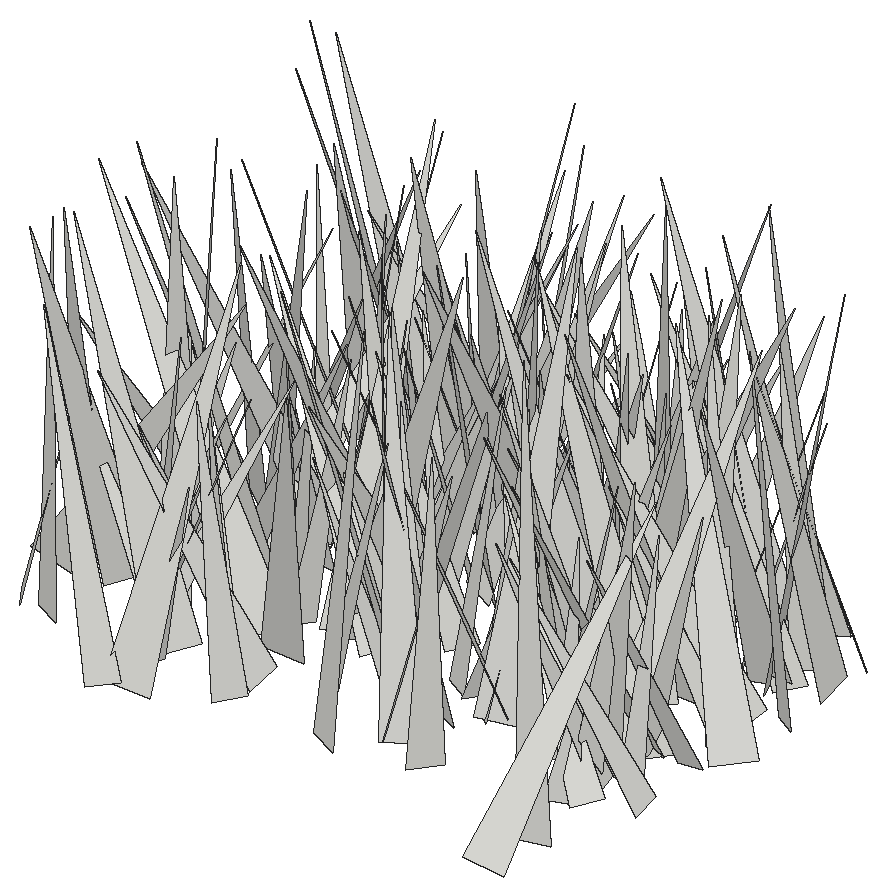
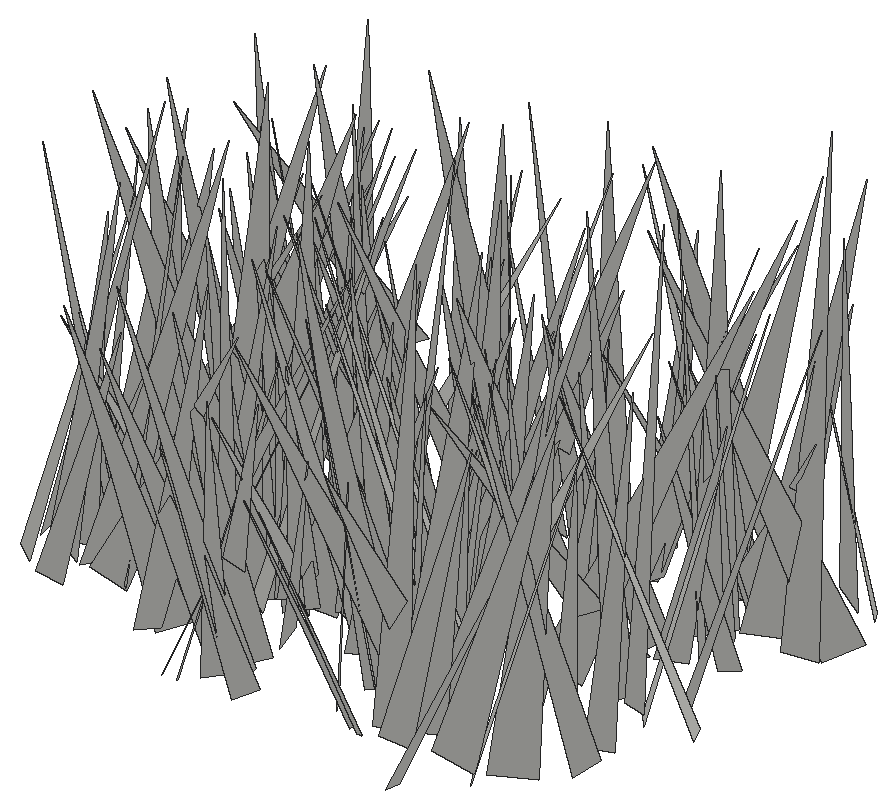
# SketchUp Ruby script. Lengths in inches.
U = 1.inch
M = Sketchup.active_model
def pt(a) = Geom::Point3d.new(a.map { |v| v * U })
def face(e, loops, mat)
  f = e.add_face(loops[0].map { |a| pt(a) })
  loops[1..].each { |l| e.add_face(l.map { |a| pt(a) }).erase! }
  f.material = f.back_material = mat if mat
  f
end
# faces: each face lists its corners as indices into pts; further lists are holes
def faces(e, pts, list, mat = nil) = list.each { |f| face(e, (f[0].is_a?(Array) ? f : [f]).map { |l| l.map { |i| pts[i] } }, mat) }
# xy, xz, yz: faces in a plane at the given z, y or x. An outline is a flat list of corners, or four numbers for a rectangle; further outlines are holes
def ring(l) = l.size == 4 ? [[l[0], l[1]], [l[2], l[1]], [l[2], l[3]], [l[0], l[3]]] : l.each_slice(2).to_a
def flat(e, list, mat, &to3) = list.each { |f| face(e, (f[0].is_a?(Array) ? f : [f]).map { |l| ring(l).map { |u, v| to3.(u, v) } }, mat) }
def xy(e, z, list, mat = nil) = flat(e, list, mat) { |x, y| [x, y, z] }
def xz(e, y, list, mat = nil) = flat(e, list, mat) { |x, z| [x, y, z] }
def yz(e, x, list, mat = nil) = flat(e, list, mat) { |y, z| [x, y, z] }
def lines(e, pts, list) = list.each { |a, b| e.add_line(pt(pts[a]), pt(pts[b])) }
# prism: a flat outline (further loops are holes) pulled along v
def prism(e, loops, v, mat = nil)
  f = face(e, loops, mat); d = Geom::Vector3d.new(v.map { |x| x * U })
  f.pushpull(f.normal.samedirection?(d) ? d.length : -d.length)
end
def box(e, o, s, mat = nil) = prism(e, [[o, [o[0] + s[0], o[1], o[2]], [o[0] + s[0], o[1] + s[1], o[2]], [o[0], o[1] + s[1], o[2]]]], [0, 0, s[2]], mat)
def at(x, y, z, deg = 0) = Geom::Transformation.translation(pt([x, y, z])) * Geom::Transformation.rotation(ORIGIN, Z_AXIS, deg.degrees)
def axes(o, x, y, z) = Geom::Transformation.new([*x, 0, *y, 0, *z, 0, *pt(o).to_a, 1])
def part(name) = M.definitions.add(name)
# library, detail: a bought-in or finely detailed component or shape, given as its bounding box
def library(name, o, s) = part(name).tap { |d| box(d.entities, o, s) }
def detail(e, o, s) = box(e.add_group.entities, o, s)
def put(e, d, t, mat = nil) = e.add_instance(d, t).tap { |i| i.material = mat if mat }
def group(e, t, mat = nil) = e.add_group.tap { |g| g.transformation = t; g.material = mat if mat }.entities
root = M.entities
c1 = part("fur_instance\#9")
p = [[0.8125,0,1.79],[0.67,-0.02,1.48],[0,-0.11,0],[0,0.11,0]]
faces(c1.entities,p,[[0,1,2,3]])
put(root,c1,axes([93.54,413.52,-27.1],[-1.50811,5.89701,0.63499],[5.61901,1.21081,2.10069],[-1.89858,-1.1007,5.71281]))
put(root,c1,axes([110.04,411.91,-27.1],[-2.9172,5.75801,0.16061],[5.28877,2.74872,-2.48273],[2.2824,0.99014,5.95825]))
put(root,c1,axes([97.21,415.26,-27.1],[-4.02078,2.93374,1.78068],[3.22926,4.16274,0.43339],[1.1617,-1.41743,4.95839]))
put(root,c1,axes([93.89,415.61,-27.1],[3.66443,-1.25509,0.51627],[-1.25966,-3.69872,-0.05095],[-0.50503,0.11865,3.87307]))
put(root,c1,axes([94.28,413.79,-27.1],[-1.25446,7.26591,1.58891],[7.27727,1.53186,-1.25954],[1.53602,-1.32352,7.26503]))
put(root,c1,axes([104.67,415.7,-27.1],[4.30224,-3.16543,2.15858],[-3.43037,-4.62804,0.05027],[-1.70646,1.32286,5.34104]))
put(root,c1,axes([97.22,416.94,-27.1],[-5.99784,0.36822,0.31916],[0.44096,5.77868,1.61988],[0.20737,-1.63795,5.78668]))
put(root,c1,axes([110.3,414.05,-27.1],[0.70044,7.59304,1.85976],[7.56257,-1.13109,1.76971],[-1.98005,-1.63401,7.41708]))
put(root,c1,axes([93.37,414.75,-27.1],[3.56009,0.21869,0.65734],[0.01468,-3.46445,1.07311],[-0.69261,1.05069,3.40155]))
put(root,c1,axes([101.21,414.95,-27.1],[3.25616,5.95918,2.11371],[6.15078,-3.5363,0.49462],[-1.46542,-1.60155,6.77272]))
put(root,c1,axes([88.04,416.32,-27.1],[3.15545,2.01724,0.79775],[2.15051,-3.09372,-0.68323],[-0.2846,-1.01105,3.6823]))
put(root,c1,axes([93.95,416.64,-27.1],[-6.02527,4.37662,1.94606],[4.73834,5.90349,1.39383],[0.70004,-2.28907,7.31546]))
put(root,c1,axes([96.71,418.52,-27.1],[1.84605,-6.6162,0.27609],[-6.51912,-1.76548,1.28157],[1.16252,0.60597,6.74831]))
put(root,c1,axes([92.05,418.23,-27.1],[6.81977,1.54998,0.06465],[1.44583,-6.24479,-2.79788],[0.56233,-2.74155,6.40965]))
put(root,c1,axes([102.37,416.625,-27.1],[3.27913,1.40298,0.59687],[1.4938,-3.23974,-0.59158],[-0.30522,-0.78299,3.51725]))
put(root,c1,axes([89.36,415.97,-27.1],[3.04497,5.63186,2.55497],[5.93211,-3.46487,0.56775],[-1.7481,-1.94792,6.3771]))
put(root,c1,axes([111.65,418.02,-27.1],[-4.90231,-0.23018,0.15933],[-0.18525,4.76264,1.18065],[0.20988,-1.17272,4.76358]))
put(root,c1,axes([109.8125,418.23,-27.1],[-4.7933,-0.97536,0.74224],[-0.77682,4.73507,1.20565],[0.94805,-1.05153,4.74061]))
put(root,c1,axes([95.92,416.74,-27.1],[-4.49863,-0.46507,1.40367],[-0.60193,4.68178,-0.37796],[1.35065,0.53749,4.50678]))
put(root,c1,axes([89.95,419.36,-27.1],[5.20163,-5.29224,1.8402],[-4.95757,-5.51713,-1.85336],[-2.61089,-0.0677,7.18539]))
put(root,c1,axes([94.8,418.69,-27.1],[-4.25051,-1.02119,0.70994],[-0.79222,4.17184,1.25768],[0.95876,-1.08007,4.18663]))
put(root,c1,axes([88.28,419.73,-27.1],[-1.25565,-8.18969,1.33935],[-8.04493,1.53362,1.83538],[2.03567,1.00923,8.07955]))
put(root,c1,axes([103.15,416.48,-27.1],[-2.95923,6.17255,1.7602],[6.41346,2.92118,0.53848],[0.25723,-1.82266,6.82403]))
put(root,c1,axes([103.28,418.46,-27.1],[-2.87551,-4.98025,1.4124],[-5.17006,2.84441,-0.49611],[0.26119,1.47404,5.72934]))
put(root,c1,axes([98.9,418.29,-27.1],[3.06956,3.90435,1.71137],[4.25532,-2.68017,-1.51785],[0.25498,-2.27325,4.72887]))
put(root,c1,axes([110.06,417.07,-27.1],[-3.00277,4.1066,0.06153],[3.92812,2.84936,1.52829],[-1.19912,-0.94951,4.85234]))
put(root,c1,axes([109.02,419.01,-27.1],[1.26894,-6.32164,1.3833],[-6.3592,-0.957,1.46001],[1.19887,1.6149,6.28026]))
put(root,c1,axes([109.34,417.8,-27.1],[4.20018,-2.603,1.54886],[-2.85846,-4.28223,0.55487],[-1.0019,1.30501,4.91012]))
put(root,c1,axes([92.45,417.33,-27.1],[4.52412,1.43506,1.852],[1.32361,-4.8885,0.5546],[-1.93323,0.01133,4.71375]))
put(root,c1,axes([92.18,418.05,-27.1],[-2.52559,2.65872,0.46687],[2.62617,2.27215,1.26725],[-0.62447,-1.19747,3.44114]))
put(root,c1,axes([95.65,417.19,-27.1],[-3.44021,1.49763,0.22694],[1.46636,3.43395,-0.43273],[0.37973,0.30751,3.72702]))
put(root,c1,axes([107.625,419.05,-27.1],[-1.75963,-5.21212,1.71135],[-5.46295,1.82898,-0.04671],[0.50104,1.63703,5.50093]))
put(root,c1,axes([101.33,418.78,-27.1],[-5.74367,-4.09689,1.01684],[-4.21686,5.6466,-1.0688],[0.19121,1.46278,6.97366]))
put(root,c1,axes([109.2,416.54,-27.1],[-3.77654,1.99621,0.89861],[1.50689,3.67022,-1.82025],[1.58796,1.26459,3.86442]))
put(root,c1,axes([87.36,418.74,-27.1],[3.63581,-6.29578,1.08718],[-5.74464,-2.67402,3.72648],[2.79605,2.69271,6.24254]))
put(root,c1,axes([90.93,418.79,-27.1],[2.90459,3.11145,0.76807],[3.13189,-2.53582,-1.57117],[0.67994,-1.61126,3.9559]))
put(root,c1,axes([107.38,418.88,-27.1],[4.01593,3.70117,1.52807],[3.99587,-3.8439,-1.19115],[-0.25835,-1.92018,5.32987]))
put(root,c1,axes([109.5,420.9375,-27.1],[-1.38983,-5.84462,0.0201],[-5.82782,1.38425,-0.46046],[-0.44334,0.12603,5.98992]))
put(root,c1,axes([107.8,418.7,-27.1],[0.95056,-3.70171,1.6828],[-4.06505,-0.90725,0.30052],[-0.09921,1.70654,3.80998]))
put(root,c1,axes([92.52,417.35,-27.1],[1.65691,4.63189,0.02775],[4.518,-1.60961,-1.09423],[1.0212,-0.39403,4.79608]))
put(root,c1,axes([100.51,419.1875,-27.1],[-3.97846,-0.22397,0.26493],[-0.21326,3.98441,0.16592],[0.27363,-0.15114,3.9813]))
put(root,c1,axes([101.83,419.15,-27.1],[-1.39517,3.65073,1.37856],[3.73252,0.82124,1.60268],[-1.13865,-1.78115,3.56451]))
put(root,c1,axes([95.36,419.24,-27.1],[-7.15301,3.97515,0.71331],[4.02795,6.91641,1.848],[-0.2937,-1.95899,7.97197]))
put(root,c1,axes([111.08,420.95,-27.1],[-0.25255,-4.7231,0.0991],[-4.68784,0.23828,-0.59045],[-0.58449,0.12972,4.69284]))
put(root,c1,axes([110.53,418.67,-27.1],[0.04059,4.23783,1.33242],[4.44047,0.00019,-0.13586],[0.12965,-1.33303,4.23585]))
put(root,c1,axes([107.43,417.43,-27.1],[1.37607,4.21587,0.41156],[3.82506,-1.42264,1.78368],[-1.81985,0.19763,4.06025]))
put(root,c1,axes([104.52,419.98,-27.1],[-5.23491,-4.53939,0.15815],[-4.43832,5.06084,-1.65066],[-0.96564,1.34804,6.72946]))
put(root,c1,axes([101.74,418.95,-27.1],[-4.02288,2.74208,1.38872],[2.85785,4.17888,0.02734],[1.13147,-0.80565,4.86845]))
put(root,c1,axes([106.97,420.83,-27.1],[3.89618,-1.88557,1.1779],[-1.51971,-3.99347,-1.36592],[-1.62275,-0.78732,4.1073]))
put(root,c1,axes([91.29,420.26,-27.1],[6.49174,-3.69034,2.54193],[-3.75607,-6.92147,-0.45599],[-2.44375,0.83512,7.45341]))
put(root,c1,axes([108.35,420.47,-27.1],[-6.30832,-1.1114,1.05664],[-1.00602,6.37534,0.69964],[1.15742,-0.51611,6.36715]))
put(root,c1,axes([92.85,418.13,-27.1],[-4.63028,1.37895,0.71291],[1.15549,4.55932,-1.31404],[1.03661,1.07721,4.64912]))
put(root,c1,axes([108.73,420.92,-27.1],[-1.67937,-5.43767,0.87836],[-5.25266,1.30456,-1.96667],[-1.65811,1.37475,5.34049]))
put(root,c1,axes([99.68,420.62,-27.1],[3.13596,-3.23192,0.2957],[-3.22644,-3.06024,0.76944],[0.35051,0.74607,4.43707]))
put(root,c1,axes([97.97,420.8,-27.1],[6.25642,-5.32962,1.03257],[-5.42827,-6.12142,1.29455],[0.06986,1.65444,8.11614]))
put(root,c1,axes([98.69,423.33,-27.1],[5.3138,-2.81187,1.14067],[-1.98861,-4.96443,-2.9739],[-2.29198,-2.2118,5.22484]))
put(root,c1,axes([104.12,419.29,-27.1],[2.60004,3.22909,0.64132],[3.22546,-2.66223,0.32783],[-0.65933,-0.2899,4.13277]))
put(root,c1,axes([98.32,422.99,-27.1],[-0.28332,-7.79704,0.77926],[-7.68212,0.12267,-1.56569],[-1.54472,0.82004,7.64347]))
put(root,c1,axes([109.55,420.5,-27.1],[4.23339,-1.74729,1.15695],[-1.93705,-4.25778,0.65751],[-0.79963,1.0637,4.53236]))
put(root,c1,axes([99.19,420.59,-27.1],[4.97701,4.02381,2.97396],[4.34378,-5.5566,0.24873],[-2.48337,-1.65505,6.3953]))
put(root,c1,axes([94.78,420.7,-27.1],[-7.32124,-3.15954,0.71739],[-3.23761,7.2018,-1.32279],[0.12329,1.49974,7.86343]))
put(root,c1,axes([95.95,420.41,-27.1],[4.38322,-1.64948,1.59394],[-1.93146,-4.50849,0.64578],[-1.2373,1.19448,4.63858]))
put(root,c1,axes([104.78,419.4,-27.1],[-2.78975,7.45432,2.27613],[7.61508,3.12201,-0.8911],[1.66081,-1.79348,7.90921]))
put(root,c1,axes([105.29,420.04,-27.1],[-1.61358,3.38665,0.61033],[3.4322,1.63258,0.01498],[0.24881,-0.55751,3.75138]))
put(root,c1,axes([88.97,424.53,-27.1],[-5.2943,-3.28141,1.0592],[-2.29433,4.80125,3.40634],[2.57403,-2.46971,5.21479]))
put(root,c1,axes([102.29,420.25,-27.1],[2.52877,4.50107,1.40807],[4.66336,-2.62485,0.01569],[-0.70386,-1.21962,5.16276]))
put(root,c1,axes([102.89,421.92,-27.1],[3.51068,-4.45404,1.06123],[-4.56743,-3.50052,0.41776],[-0.32136,1.09429,5.65587]))
put(root,c1,axes([99.51,421.69,-27.1],[1.40139,-5.88916,2.09043],[-6.21682,-1.53152,-0.14692],[-0.635,1.99706,6.05182]))
put(root,c1,axes([103.08,420.1875,-27.1],[5.00649,-0.69371,1.01239],[-0.92226,-4.93206,1.18126],[-0.80969,1.32843,4.91435]))
put(root,c1,axes([98.99,420.67,-27.1],[-4.99082,4.3261,0.4502],[4.29852,4.80129,1.51542],[-0.66378,-1.43477,6.4286]))
put(root,c1,axes([94.99,421.5,-27.1],[-3.86454,-2.68359,1.87384],[-2.96857,4.09497,-0.25773],[1.3786,1.29506,4.69786]))
put(root,c1,axes([109.89,420.72,-27.1],[-2.9065,7.574,1.65107],[7.44857,2.24028,2.83534],[-2.14716,-2.4809,7.60092]))
put(root,c1,axes([90.45,421.83,-27.1],[6.26613,3.81902,2.82967],[4.24719,-6.60086,-0.4964],[-2.13385,-1.92357,7.3214]))
put(root,c1,axes([90.23,420.76,-27.1],[-4.86729,-1.78674,2.25978],[-2.35287,5.02555,-1.09424],[1.66225,1.88173,5.06809]))
put(root,c1,axes([94.93,421.37,-27.1],[4.11345,0.18865,1.81103],[0.00918,-4.47631,0.44541],[-1.8208,0.4036,4.09361]))
put(root,c1,axes([89.45,421.75,-27.1],[0.33455,3.97904,1.71347],[4.11253,0.24873,-1.38056],[1.36232,-1.72801,3.74683]))
put(root,c1,axes([92.24,421.9375,-27.1],[4.93305,-2.19664,0.15391],[-2.18894,-4.85066,0.92924],[0.23965,0.9109,5.31946]))
put(root,c1,axes([108.61,424.14,-27.1],[-0.93689,-7.58778,0.99671],[-7.63501,0.85799,-0.64504],[-0.52389,1.06539,7.61814]))
put(root,c1,axes([100.84,422.375,-27.1],[-3.29735,3.76242,1.32483],[3.9802,2.99017,1.41439],[-0.2628,-1.92005,4.79874]))
put(root,c1,axes([110.91,422.9,-27.1],[-4.62797,0.36048,0.06702],[0.36662,4.56134,0.78248],[0.00509,-0.78533,4.57556]))
put(root,c1,axes([108.73,419.96,-27.1],[-1.75958,6.89289,0.89816],[6.66639,1.93582,-1.79628],[1.96924,-0.39424,6.88342]))
put(root,c1,axes([100.51,419.7,-27.1],[7.12647,2.20024,1.82821],[1.44023,-6.99989,2.8102],[-2.47167,2.26505,6.90872]))
put(root,c1,axes([106.92,422.46,-27.1],[-8.06825,0.70999,0.37952],[0.71569,8.07597,0.10667],[0.36866,-0.13964,8.09873]))
put(root,c1,axes([94.24,423.71,-27.1],[-0.05824,-3.81958,0.55077],[-3.85535,0.08183,0.15984],[0.16986,0.54776,3.81668]))
put(root,c1,axes([102.33,423.4,-27.1],[7.07527,1.73735,2.55738],[2.12787,-7.36989,-0.88027],[-2.24293,-1.5114,7.23207]))
put(root,c1,axes([91.21,422.44,-27.1],[-3.33055,3.67395,0.98734],[3.8043,3.21801,0.85849],[0.0046,-1.30837,4.884]))
put(root,c1,axes([103.05,422.7,-27.1],[1.88047,-2.78184,1.95652],[-3.20631,-2.19563,-0.04014],[-1.13412,1.59479,3.35756]))
put(root,c1,axes([112.04,421.89,-27.1],[-4.84886,5.21937,0.60309],[5.25064,4.78392,0.8135],[-0.19034,-0.99462,7.07753]))
put(root,c1,axes([110.8,424.27,-27.1],[-6.49837,1.01991,0.13564],[1.01971,6.26851,1.71854],[-0.13717,-1.71841,6.34946]))
put(root,c1,axes([104.99,423.11,-27.1],[4.67154,-2.82363,0.84685],[-2.94301,-4.55853,1.0353],[-0.16964,1.32674,5.35951]))
put(root,c1,axes([93.52,425.01,-27.1],[0.24896,-7.3468,1.55373],[-6.97419,-0.80255,-2.67734],[-2.78393,1.35351,6.84612]))
put(root,c1,axes([104.75,425.08,-27.1],[-0.95692,-4.60949,0.0097],[-4.59629,0.95343,-0.35816],[-0.34872,0.08227,4.69412]))
put(root,c1,axes([89.56,425.88,-27.1],[-5.06426,-4.56399,0.84014],[-4.29824,5.08189,1.69768],[1.74956,-0.72593,6.60262]))
put(root,c1,axes([102.01,426.72,-27.1],[1.8393,-7.94223,0.20343],[-7.82957,-1.84746,-1.33722],[-1.34842,-0.10629,8.04201]))
put(root,c1,axes([90.24,425.47,-27.1],[-3.33298,-6.74445,1.96036],[-6.484,3.7887,2.01069],[2.69971,0.77298,7.24938]))
put(root,c1,axes([99.2,425.76,-27.1],[-3.9717,-6.10655,1.7462],[-5.81347,4.32471,1.90107],[2.55787,0.34722,7.03209]))
put(root,c1,axes([107.67,423.125,-27.1],[-5.36752,5.77658,2.45123],[6.12108,5.53013,0.37117],[1.38195,-2.05828,7.87664]))
put(root,c1,axes([98.78,423.57,-27.1],[-0.11529,-4.79427,2.44231],[-5.06003,0.9271,1.58106],[1.8292,2.26244,4.52754]))
put(root,c1,axes([90.97,425.34,-27.1],[7.66875,0.29762,1.40281],[0.64374,-7.5341,-1.92071],[-1.28143,-2.00373,7.43029]))
put(root,c1,axes([102.77,421.22,-27.1],[3.19327,6.60837,0.52108],[6.51338,-3.23542,1.11669],[-1.23207,0.02336,7.254]))
put(root,c1,axes([95.83,423.9,-27.1],[3.79573,2.84609,1.46317],[3.05532,-3.89817,-0.34352],[-0.95191,-1.16307,4.73179]))
put(root,c1,axes([111.21,422.53,-27.1],[-0.8728,6.82324,1.17968],[6.78553,0.6058,1.51645],[-1.38016,-1.33658,6.7096]))
put(root,c1,axes([109.79,426.58,-27.1],[2.0561,-6.44135,0.2848],[-6.4395,-2.06652,-0.24899],[-0.32395,0.19535,6.75697]))
put(root,c1,axes([105.97,424.36,-27.1],[7.40162,-2.04644,1.37858],[-2.14984,-7.48787,0.42713],[-1.21103,0.78507,7.66743]))
put(root,c1,axes([101.21,426.48,-27.1],[0.94954,-6.1364,0.24208],[-6.03443,-0.88683,1.18943],[1.14,0.41683,6.09444]))
put(root,c1,axes([96.5,424.83,-27.1],[-4.53938,3.59005,2.40826],[4.08452,4.7056,0.68422],[1.41595,-2.06469,5.74685]))
put(root,c1,axes([96.81,424.44,-27.1],[-5.69424,-4.56861,0.52497],[-4.47673,5.31586,-2.29625],[-1.05201,2.10752,6.92992]))
put(root,c1,axes([103.17,426.95,-27.1],[-1.64763,-7.14584,1.34901],[-6.49832,2.06763,3.01567],[3.26416,0.50931,6.68457]))
put(root,c1,axes([99.08,425.26,-27.1],[-3.66395,-2.75565,0.79106],[-2.79858,3.7164,-0.01609],[0.62239,0.48852,4.58453]))
put(root,c1,axes([97.39,420.81,-27.1],[-7.03666,4.34174,0.35439],[3.96979,6.66848,-2.87454],[1.79361,2.2741,7.75256]))
put(root,c1,axes([102.15,427.02,-27.1],[0.44147,-7.17503,0.62576],[-6.54369,-0.13768,3.03788],[3.00878,0.75334,6.51516]))
put(root,c1,axes([103.5,426.67,-27.1],[2.17041,-4.52553,0.56409],[-4.42394,-2.24099,-0.95709],[-1.10786,0.0828,4.92697]))
put(root,c1,axes([106.53,425.3,-27.1],[-5.73495,-0.11109,1.68244],[-0.04447,5.97258,0.24275],[1.68552,-0.22038,5.73089]))
put(root,c1,axes([111.72,424.86,-27.1],[-3.6941,-4.73944,2.34113],[-5.23892,3.66336,-0.85037],[0.70493,2.38895,5.94858]))
put(root,c1,axes([108.33,424.79,-27.1],[4.86014,-4.74094,2.82615],[-5.30574,-5.05065,0.65171],[-1.52079,2.46963,6.75816]))
put(root,c1,axes([101.46,424.8,-27.1],[-3.65531,3.57205,1.42816],[3.77376,3.712,0.37448],[0.74692,-1.27356,5.09712]))
put(root,c1,axes([102.6,426.45,-27.1],[4.53182,-5.76132,1.66498],[-5.89155,-4.66684,-0.11276],[-1.12014,1.237,7.32923]))
put(root,c1,axes([103.43,427.58,-27.1],[-4.06699,-5.2197,0.56162],[-5.13541,4.10303,0.94539],[1.09007,-0.14467,6.54919]))
put(root,c1,axes([95.58,423.93,-27.1],[-5.55203,-0.57439,2.02149],[-1.15794,5.60149,-1.58866],[1.75372,1.88009,5.3508]))
put(root,c1,axes([97.56,424.86,-27.1],[-5.21816,-1.76906,1.50642],[-2.07355,5.2165,-1.05669],[1.04846,1.51216,5.4076]))
put(root,c1,axes([104.67,426.67,-27.1],[1.53942,-5.44162,0.89342],[-5.38829,-1.28703,1.44538],[1.17292,1.22946,5.46735]))
put(root,c1,axes([98.83,428.02,-27.1],[4.29462,-4.11505,0.26594],[-3.98176,-4.23808,-1.27765],[-1.07236,-0.74374,5.80905]))
put(root,c1,axes([87.69,425.57,-27.1],[5.0651,3.0377,0.15182],[3.00547,-4.95362,-1.15532],[0.46672,-1.0677,5.79207]))
put(root,c1,axes([100.43,426.71,-27.1],[-1.57238,-4.56901,1.11948],[-4.65933,1.35009,-1.0341],[-0.64787,1.37945,4.72005]))
put(root,c1,axes([89.45,428.2,-27.1],[-0.0268,-5.65268,0.22398],[-5.53849,0.07185,1.15049],[1.15241,0.21383,5.53443]))
put(root,c1,axes([103.93,426.76,-27.1],[6.6749,-4.96789,0.00129],[-4.8195,-6.47499,2.02019],[1.20515,1.62135,8.07174]))
put(root,c1,axes([92.21,423.23,-27.1],[-1.93127,6.17376,0.09606],[5.65668,1.80943,-2.5656],[2.47519,0.68189,5.93825]))
put(root,c1,axes([96.31,426.62,-27.1],[3.07396,-3.53335,0.83024],[-3.61315,-2.87553,1.13994],[0.34489,1.36741,4.5425]))
put(root,c1,axes([110.48,426.6875,-27.1],[-2.9134,4.03937,1.46912],[4.26943,2.51447,1.5531],[-0.49677,-2.07934,4.73205]))
put(root,c1,axes([94.87,427.2,-27.1],[7.11507,4.33314,0.48127],[4.20256,-6.57141,-2.9643],[1.16029,-2.76992,7.78545]))
put(root,c1,axes([111.57,427.5,-27.1],[-7.78363,-1.77881,1.5879],[-1.77027,7.9428,0.22014],[1.59741,0.13482,7.98126]))
put(root,c1,axes([108.25,427.13,-27.1],[4.56554,2.4835,0.72557],[2.58092,-4.47494,-0.92307],[-0.18188,-1.15993,5.11467]))
put(root,c1,axes([96.28,427.02,-27.1],[1.74245,-3.02379,2.07472],[-3.3962,-2.19711,-0.34987],[-1.38332,1.58534,3.47232]))
put(root,c1,axes([98.14,427.5,-27.1],[-0.07815,-6.05054,2.52953],[-6.4447,0.53908,1.09033],[1.2138,2.47266,5.952]))
put(root,c1,axes([102.42,426.51,-27.1],[-3.32764,3.062,1.30373],[3.08153,3.53122,-0.42827],[1.25687,-0.55083,4.50173]))
put(root,c1,axes([92.98,426.41,-27.1],[4.79862,3.05458,1.6678],[3.017,-5.06719,0.60002],[-1.73486,-0.36311,5.65661]))
put(root,c1,axes([109.79,426.53,-27.1],[6.18065,2.99725,1.89028],[2.99834,-6.44896,0.42186],[-1.88855,-0.42956,6.85609]))
put(root,c1,axes([104.9,427.9,-27.1],[-2.89308,-3.13599,0.85003],[-3.23039,2.89836,-0.3018],[0.34876,0.83187,4.25597]))
put(root,c1,axes([108.58,424.99,-27.1],[4.22042,3.02936,0.44277],[2.70703,-4.0447,1.87014],[-1.43005,1.2839,4.84681]))
put(root,c1,axes([105.48,428.98,-27.1],[-6.50951,0.22142,0.60358],[0.38251,6.26967,1.82536],[0.51674,-1.85181,6.25226]))
put(root,c1,axes([93.46,425.1,-27.1],[5.52585,4.05046,1.31825],[3.69086,-5.63091,1.83015],[-2.12639,0.75214,6.60241]))
put(root,c1,axes([97.21,428.14,-27.1],[2.58883,2.26123,2.35644],[2.87323,-3.00647,-0.27159],[-1.55259,-1.79333,3.42658]))
put(root,c1,axes([99.04,425.39,-27.1],[3.08355,6.47581,0.56476],[6.50039,-3.07095,-0.27862],[0.00972,-0.62967,7.16706]))
put(root,c1,axes([97.79,425.65,-27.1],[6.38887,5.18246,1.59043],[5.07791,-6.58181,1.04866],[-1.89794,-0.16426,8.1594]))
put(root,c1,axes([111.0625,429.53,-27.1],[-3.86726,-4.8383,0.71579],[-4.78645,3.93151,0.71436],[1.00566,0.10641,6.1526]))
put(root,c1,axes([110.19,428.03,-27.1],[1.93856,-5.12728,2.24723],[-5.46022,-2.25638,-0.43794],[-1.23493,1.9279,5.46399]))
put(root,c1,axes([107.72,428.86,-27.1],[4.54557,4.08977,3.87164],[5.12111,-5.0718,-0.65499],[-2.34307,-3.15097,6.07942]))
put(root,c1,axes([99.33,427.37,-27.1],[6.39922,1.66084,0.77373],[1.68967,-6.43637,-0.15871],[-0.70856,-0.34898,6.60932]))
put(root,c1,axes([94.66,429.43,-27.1],[-4.58981,-6.81856,1.14154],[-6.9132,4.53833,-0.68805],[0.05895,1.33156,8.19058]))
put(root,c1,axes([92.05,426.58,-27.1],[1.02305,5.31057,1.33507],[5.15193,-1.39366,1.59576],[-1.8553,-0.94167,5.16743]))
put(root,c1,axes([108.83,428.37,-27.1],[-7.81883,2.51294,1.68172],[2.76611,7.82758,1.16397],[1.22135,-1.64052,8.12983]))
put(root,c1,axes([96.57,429.13,-27.1],[-2.51428,-3.3921,0.48717],[-3.39486,2.54791,0.21985],[0.4675,0.25907,4.21659]))
put(root,c1,axes([94.82,428.4,-27.1],[6.0574,2.72005,0.2303],[2.69232,-5.86042,-1.5971],[0.45071,-1.54939,6.44516]))
put(root,c1,axes([94.48,430.8,-27.1],[5.05065,-5.78899,0.88016],[-5.66798,-5.12516,-1.18448],[-1.47008,-0.1285,7.59069]))
put(root,c1,axes([96.73,428.47,-27.1],[4.08139,-3.20586,0.61223],[-3.2526,-3.91407,1.18774],[0.27008,1.30866,5.05219]))
put(root,c1,axes([96.99,429.28,-27.1],[1.53835,-7.01276,2.03333],[-7.04829,-0.88366,2.28484],[1.90652,2.39168,6.80623]))
put(root,c1,axes([96,429.28,-27.1],[-2.86919,-3.90872,1.79506],[-4.01549,3.2075,0.56601],[1.54149,1.08002,4.8156]))
put(root,c1,axes([90.48,431.18,-27.1],[4.1786,-6.03386,0.40804],[-6.0035,-4.19846,-0.60465],[-0.72937,-0.01047,7.31455]))
put(root,c1,axes([102.89,429.67,-27.1],[7.08469,1.17747,2.52447],[1.61288,-7.35894,-1.094],[-2.27113,-1.55299,7.09806]))
put(root,c1,axes([91.4,430.97,-27.1],[-2.96228,-3.48582,0.87467],[-2.85625,2.97145,2.16874],[2.18125,-0.843,4.02773]))
put(root,c1,axes([102.74,429.43,-27.1],[3.92592,-0.41216,0.89749],[-0.2951,-4.00034,-0.54626],[-0.94248,-0.46433,3.90952]))
put(root,c1,axes([110.44,428.39,-27.1],[1.97558,6.78512,3.04566],[6.89111,-2.85534,1.89119],[-2.79761,-2.24188,6.80913]))
put(root,c1,axes([102.38,426.31,-27.1],[4.15865,3.49208,0.81847],[2.77358,-3.92559,2.6563],[-2.27416,1.59814,4.73636]))
put(root,c1,axes([95.24,431.23,-27.1],[-0.53699,-7.34105,1.16615],[-7.27133,0.76139,1.44476],[1.5423,1.0337,7.21748]))
put(root,c1,axes([89,429.37,-27.1],[6.32916,0.13104,0.27334],[0.13733,-6.3333,-0.14369],[-0.27023,-0.14945,6.32889]))
put(root,c1,axes([108.02,429.2,-27.1],[-2.44299,5.49091,1.30941],[5.27932,1.71736,2.64808],[-1.99837,-2.17564,5.395]))
put(root,c1,axes([109.48,430.3,-27.1],[0.38107,-4.3176,1.24457],[-4.35966,-0.65774,-0.94692],[-1.08815,1.12319,4.22969]))
put(root,c1,axes([101.37,428.66,-27.1],[-4.4304,-0.23548,0.66281],[-0.42328,4.26855,-1.31284],[0.56178,1.35914,4.23796]))
put(root,c1,axes([101.25,430.52,-27.1],[4.31446,-3.71791,0.40504],[-3.72385,-4.21342,0.9907],[0.3462,1.01276,5.60856]))
put(root,c1,axes([97.84,428.84,-27.1],[-4.49953,-3.59508,3.80394],[-4.60675,5.10137,-0.62788],[2.48443,2.94818,5.72505]))
put(root,c1,axes([104.97,430.76,-27.1],[4.62611,-3.05223,2.53258],[-2.97331,-5.24406,-0.88892],[-2.62479,0.5609,5.47054]))
put(root,c1,axes([102.95,429.93,-27.1],[1.4221,-3.78822,2.5832],[-4.25079,-2.10312,-0.74405],[-1.71882,2.06693,3.97736]))
put(root,c1,axes([103.09,432.61,-27.1],[-4.66281,-2.88259,0.04543],[-2.761,4.48988,1.50703],[0.82963,-1.25893,5.27068]))
put(root,c1,axes([95.04,429.53,-27.1],[6.3813,-2.25892,0.20905],[-2.20352,-6.02357,2.17449],[0.53935,2.11689,6.41056]))
put(root,c1,axes([102.64,430.36,-27.1],[3.58397,-3.64133,0.7361],[-3.60405,-3.15993,1.91614],[0.90107,1.84433,4.7363]))
put(root,c1,axes([94.66,431.73,-27.1],[0.91416,-4.94391,1.27953],[-4.9749,-1.15567,-0.91103],[-1.1532,1.06645,4.94449]))
put(root,c1,axes([102.39,432.84,-27.1],[-3.17214,-2.54983,0.51656],[-2.07776,2.97317,1.9168],[1.56569,-1.22048,3.59026]))
put(root,c1,axes([97.56,430.97,-27.1],[2.96101,1.91002,1.7712],[2.18546,-3.28075,-0.11568],[-1.41742,-1.06838,3.5217]))
put(root,c1,axes([104.51,430.3125,-27.1],[3.63193,-4.05591,1.60644],[-4.34601,-3.18259,1.79036],[0.37856,2.37544,5.14159]))
put(root,c1,axes([95.87,428.18,-27.1],[-4.47907,3.89554,0.463],[3.44419,4.24137,-2.36643],[1.87807,1.51235,5.44401]))
put(root,c1,axes([96.32,431.77,-27.1],[2.45066,3.05169,0.44917],[2.65928,-1.79957,-2.28257],[1.56295,-1.7231,3.17938]))
put(root,c1,axes([101.59,431.92,-27.1],[3.58428,-2.61771,1.24135],[-2.70899,-3.7283,-0.04015],[-1.02701,0.69843,4.43823]))
put(root,c1,axes([92.49,431.6,-27.1],[0.18988,-6.4583,3.19895],[-6.79344,-1.22898,-2.07794],[-2.40669,2.95955,6.11783]))
put(root,c1,axes([91.7,431.5,-27.1],[-6.3033,-3.29184,1.05702],[-3.45211,6.11366,-1.54635],[0.19083,1.86335,6.94094]))
put(root,c1,axes([100.15,432.25,-27.1],[3.34433,-2.45993,0.06359],[-2.39384,-3.22746,1.0454],[0.56992,0.87868,4.01783]))
put(root,c1,axes([100.78,431.55,-27.1],[6.76067,1.19839,0.69108],[1.18973,-6.79585,0.14582],[-0.7059,0.02372,6.86451]))
put(root,c1,axes([95.84,432.04,-27.1],[2.51119,2.94201,0.30611],[2.79372,-2.22715,-1.51331],[0.97173,-1.19981,3.55969]))
put(root,c1,axes([92.99,433.96,-27.1],[-4.59731,-1.23154,0.33008],[-1.08177,4.4213,1.42926],[0.67485,-1.30242,4.53973]))
